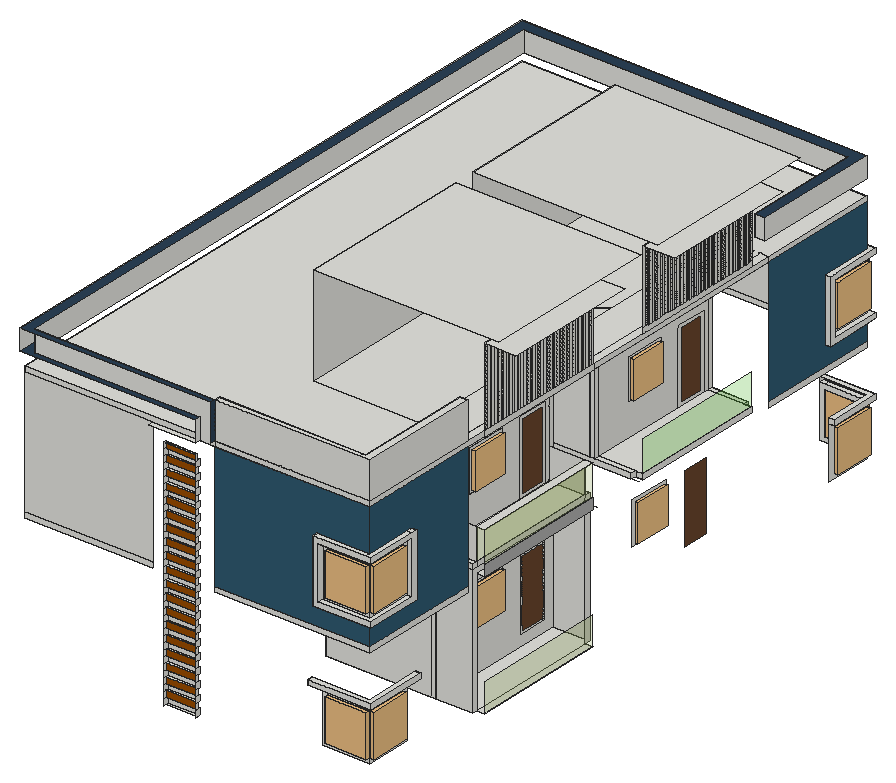
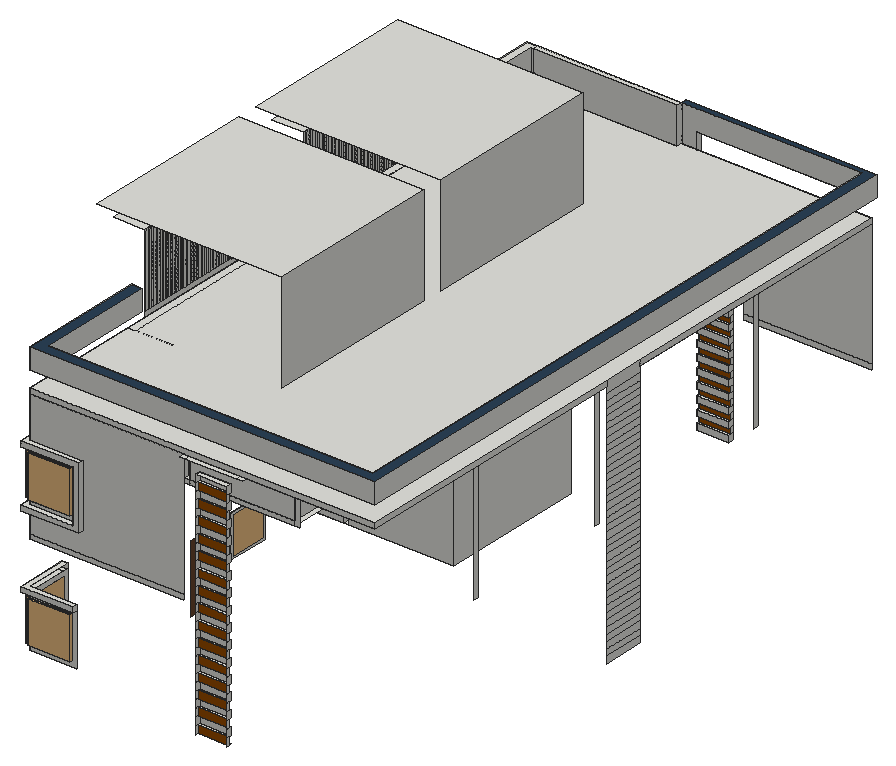
# SketchUp Ruby script. Lengths in inches.
U = 1.inch
M = Sketchup.active_model
def pt(a) = Geom::Point3d.new(a.map { |v| v * U })
def face(e, loops, mat)
  f = e.add_face(loops[0].map { |a| pt(a) })
  loops[1..].each { |l| e.add_face(l.map { |a| pt(a) }).erase! }
  f.material = f.back_material = mat if mat
  f
end
# faces: each face lists its corners as indices into pts; further lists are holes
def faces(e, pts, list, mat = nil) = list.each { |f| face(e, (f[0].is_a?(Array) ? f : [f]).map { |l| l.map { |i| pts[i] } }, mat) }
# xy, xz, yz: faces in a plane at the given z, y or x. An outline is a flat list of corners, or four numbers for a rectangle; further outlines are holes
def ring(l) = l.size == 4 ? [[l[0], l[1]], [l[2], l[1]], [l[2], l[3]], [l[0], l[3]]] : l.each_slice(2).to_a
def flat(e, list, mat, &to3) = list.each { |f| face(e, (f[0].is_a?(Array) ? f : [f]).map { |l| ring(l).map { |u, v| to3.(u, v) } }, mat) }
def xy(e, z, list, mat = nil) = flat(e, list, mat) { |x, y| [x, y, z] }
def xz(e, y, list, mat = nil) = flat(e, list, mat) { |x, z| [x, y, z] }
def yz(e, x, list, mat = nil) = flat(e, list, mat) { |y, z| [x, y, z] }
def lines(e, pts, list) = list.each { |a, b| e.add_line(pt(pts[a]), pt(pts[b])) }
# prism: a flat outline (further loops are holes) pulled along v
def prism(e, loops, v, mat = nil)
  f = face(e, loops, mat); d = Geom::Vector3d.new(v.map { |x| x * U })
  f.pushpull(f.normal.samedirection?(d) ? d.length : -d.length)
end
def box(e, o, s, mat = nil) = prism(e, [[o, [o[0] + s[0], o[1], o[2]], [o[0] + s[0], o[1] + s[1], o[2]], [o[0], o[1] + s[1], o[2]]]], [0, 0, s[2]], mat)
def at(x, y, z, deg = 0) = Geom::Transformation.translation(pt([x, y, z])) * Geom::Transformation.rotation(ORIGIN, Z_AXIS, deg.degrees)
def axes(o, x, y, z) = Geom::Transformation.new([*x, 0, *y, 0, *z, 0, *pt(o).to_a, 1])
def part(name) = M.definitions.add(name)
# library, detail: a bought-in or finely detailed component or shape, given as its bounding box
def library(name, o, s) = part(name).tap { |d| box(d.entities, o, s) }
def detail(e, o, s) = box(e.add_group.entities, o, s)
def put(e, d, t, mat = nil) = e.add_instance(d, t).tap { |i| i.material = mat if mat }
def group(e, t, mat = nil) = e.add_group.tap { |g| g.transformation = t; g.material = mat if mat }.entities
root = M.entities
M.materials.add("C07_Caramel_Shine").color = [153, 76, 0]
M.materials.add("Carpet_04_1K").color = [43, 65, 85]
M.materials.add("Glass_Basic_01").color = [173, 201, 98]
M.materials["Glass_Basic_01"].alpha = 0.25
M.materials.add("Glass_Basic_2").color = [93, 234, 42]
M.materials["Glass_Basic_2"].alpha = 0.25
M.materials.add("ThomThom - Jumper1").color = [47, 89, 112]
M.materials.add("ThomThom - Waistcoat2").color = [170, 170, 169]
M.materials.add("Wood_Veneer_15_1K").color = [103, 69, 45]
c1 = library("Group\#5",[0,0,0],[1.97,28.21,60])
xy(root,453,[[435,495,555,663],[555,495,561,663],[561,495,603,663],[603,501,612,657]])
xy(root,455.25,[[381,333,417,336]])
xy(root,458.25,[[381,1050,417,1053]])
xy(root,462.375,[[381,333,417,336]])
xy(root,467.17,[[381,1050,417,1053]])
xy(root,469.5,[[381,333,417,336]])
xy(root,476.1,[[381,1050,417,1053]])
xy(root,476.625,[[381,333,417,336]])
xy(root,483.75,[[381,333,417,336]])
xy(root,485.02,[[381,1050,417,1053]])
xy(root,490.875,[[381,333,417,336]])
xy(root,493.95,[[381,1050,417,1053]])
xy(root,498,[[381,333,417,336]])
xy(root,502.875,[[381,1050,417,1053]])
xy(root,505.125,[[381,333,417,336]])
xy(root,511.8,[[381,1050,417,1053]])
xy(root,512.25,[[381,333,417,336]])
xy(root,519.375,[[381,333,417,336]])
xy(root,520.72,[[381,1050,417,1053]])
xy(root,526.5,[[381,333,417,336]])
xy(root,529.65,[[381,1050,417,1053]])
xy(root,533.625,[[381,333,417,336]])
xy(root,534,[[546,330,558,336],[558,330,618,336],[612,336,618,390],[612,390,618,402],[612,996,618,1002],
  [612,1002,618,1056],[557.39,1050,564.01,1056],[564.01,1050,612,1056]])
xy(root,538.57,[[381,1050,417,1053]])
xy(root,540,[[546,330,618,330,618,402,612,402,612,336,546,336],[612,996,612,1050,557.39,1050,557.39,1056,618,1056,618,996]])
xy(root,540.75,[[381,333,417,336]])
xy(root,547.5,[[381,1050,417,1053]])
xy(root,547.875,[[381,333,417,336]])
xy(root,555,[[381,333,417,336]])
xy(root,556.42,[[381,1050,417,1053]])
xy(root,562.125,[[381,333,417,336]])
xy(root,565.35,[[381,1050,417,1053]])
xy(root,569.25,[[381,333,417,336]])
xy(root,574.27,[[381,1050,417,1053]])
xy(root,576.375,[[381,333,417,336]])
xy(root,583.2,[[381,1050,417,1053]])
xy(root,583.5,[[381,333,417,336]])
xy(root,590.625,[[381,333,417,336]])
xy(root,592.125,[[381,1050,417,1053]])
xy(root,593.66,[[435,723,555,891],[555,723,561,891],[561,723,603,723,603,729,612,729,612,885,603,885,603,891,561,891]])
xy(root,594,[[603,501,612,657]])
xy(root,597.75,[[381,333,417,336]])
xy(root,599.66,[[435,723,555,891],[555,723,561,891],[561,723,603,729],[561,729,612,885],[561,885,603,891]])
xy(root,600,[[435,495,555,663],[555,495,561,663],[561,495,603,663]])
xy(root,601.05,[[381,1050,417,1053]])
xy(root,602.66,[[555,846,561,876]])
xy(root,604.875,[[381,333,417,336]])
xy(root,606,[[435,495,555,663],[555,495,561,663],[561,495,603,501],[561,501,603,657],[561,657,603,663]])
xy(root,609,[[555,618,561,648]])
xy(root,609.97,[[381,1050,417,1053]])
xy(root,612,[[381,333,417,336]])
xy(root,618,[[552,330,558,336],[558,330,612,336],[612,330,618,390],[612,390,618,396],[612,990,618,1050],
  [551.39,1050,618,1056]])
xy(root,618.9,[[381,1050,417,1053]])
xy(root,619.125,[[381,333,417,336]])
xy(root,624,[[558,330,618,330,618,390,612,390,612,336,558,336],[612,996,612,1050,557.39,1050,557.39,1056,618,1056,618,996]])
xy(root,626.25,[[381,333,417,336]])
xy(root,627.83,[[381,1050,417,1053]])
xy(root,633.375,[[381,333,417,336]])
xy(root,636.75,[[381,1050,417,1053]])
xy(root,638.66,[[555,774,561,816]])
xy(root,640.5,[[381,333,417,336]])
xy(root,642,[[603,501,612,657]])
xy(root,645,[[555,546,561,588]])
xy(root,645.67,[[381,1050,417,1053]])
xy(root,647.625,[[381,333,417,336]])
xy(root,654.6,[[381,1050,417,1053]])
xy(root,654.75,[[381,333,417,336]])
xy(root,661.875,[[381,333,417,336]])
xy(root,663.52,[[381,1050,417,1053]])
xy(root,669,[[381,333,417,336]])
xy(root,672.45,[[381,1050,417,1053]])
xy(root,676.125,[[381,333,417,336]])
xy(root,680.66,[[555,774,561,816],[555,846,561,876]])
xy(root,681.375,[[381,1050,417,1053]])
xy(root,683.25,[[381,333,417,336]])
xy(root,684,[[558,330,558,336,612,336,612,390,618,390,618,330],[612,996,618,996,618,1056,557.39,1056,557.39,1050,612,1050]])
xy(root,687,[[555,546,561,588],[555,618,561,648]])
xy(root,690,[[552,330,612,336],[612,330,618,390],[612,390,618,396],[612,990,612,1050,551.39,1050,551.39,1056,618,1056,618,990]])
xy(root,690.3,[[381,1050,417,1053]])
xy(root,690.375,[[381,333,417,336]])
xy(root,697.5,[[381,333,417,336]])
xy(root,699.22,[[381,1050,417,1053]])
xy(root,704.625,[[381,333,417,336]])
xy(root,708.15,[[381,1050,417,1053]])
xy(root,711.75,[[381,333,417,336]])
xy(root,717.08,[[381,1050,417,1053]])
xy(root,718.875,[[381,332.4,417,336]])
xy(root,726,[[381,330,417,332.4],[381,1050,417,1056]])
xy(root,738,[[363,330,369,330,369,489,429,489,429,345,369,345,369,330,417,330,417,336,435,336,435,489,561,489,561,495,225,495,225,489,363,489],[216,336,363,336,363,345,225,345,225,669,216,669],[216,336,612,1050],[435,336,612,336,612,477,561,477,561,345,435,345],[429,495,435,495,435,663,555,663,555,495,561,495,561,669,225,669,225,663,429,663],
  [561,501,613,657],[216,717,216,1050,363,1050,363,1041,225,1041,225,717],[225,717,225,723,429,723,429,891,435,891,435,723,561,723,561,717],[555,723,555,891,225,891,225,897,363,897,363,1056,369,1056,369,897,429,897,429,1056,435,1056,435,897,561,897,561,723],[561,909,561,1041,435,1041,435,1050,612,1050,612,909],
  [369,1041,429,1056]])
xy(root,743.66,[[561,729,612,885]])
xy(root,744,[[216,336,612,336,612,477,602.94,477,602.94,909,612,909,612,1050,216,1050],[435,336,600,342],[600,336,600,342,603,342,603,477,612,477,612,336],[435,477,561,681],[602.94,477,612,909],
  [612,501,613,657],[435,705,561,909]])
xy(root,762,[[216,330,216,1050,612,1050,612,903.7,600,903.7,600,1038,228,1038,228,336,417,336,417,330]],"Carpet_04_1K")
xy(root,786,[[435,336,600,342],[600,336,612,336,612,477,603,477,603,342,600,342]])
xy(root,786,[[216,330,435,330,435,336,228,336,228,1038,600,1038,600,903.7,612,903.7,612,1050,216,1050]],"Carpet_04_1K")
xy(root,834,[[612,501,648,657],[612,729,648,885]])
xy(root,858,[[435,477,648,681],[435,705,648,909]])
xz(root,330,[[546,534,618,540],[552,618,618,618,618,624,558,624,558,684,618,684,618,690,552,690]])
xz(root,332.4,[[381,718.875,417,726]],"C07_Caramel_Shine")
xz(root,333,[[381,462.375,417,469.5],[381,476.625,417,483.75],[381,490.875,417,498],[381,505.125,417,512.25],[381,519.375,417,526.5],
  [381,533.625,417,540.75],[381,547.875,417,555],[381,562.125,417,569.25],[381,576.375,417,583.5],[381,590.625,417,597.75],
  [381,604.875,417,612],[381,619.125,417,626.25],[381,633.375,417,640.5],[381,647.625,417,654.75],[381,661.875,417,669],
  [381,676.125,417,683.25],[381,690.375,417,697.5],[381,704.625,417,711.75]],"C07_Caramel_Shine")
xz(root,336,[[381,455.25,417,462.375],[381,469.5,417,476.625],[558,474,612,474,612,480,564,480,564,528,612,528,612,534,558,534],[564,480,612,528],[381,483.75,417,490.875],
  [381,498,417,505.125],[381,512.25,417,519.375],[381,526.5,417,533.625],[381,540.75,417,547.875],[381,555,417,562.125],
  [381,569.25,417,576.375],[381,583.5,417,590.625],[216,588,363,594],[435,588,612,594],[216,594,363,738],
  [381,597.75,417,604.875],[381,612,417,619.125],[558,624,612,624,612,630,564,630,564,678,612,678,612,684,558,684],[381,626.25,417,633.375],[564,630,612,678],
  [381,640.5,417,647.625],[381,654.75,417,661.875],[381,669,417,676.125],[381,683.25,417,690.375],[381,697.5,417,704.625],
  [381,711.75,417,718.875],[216,738,612,744],[417,738,417,762,228,762,228,786,435,786,435,738],[435,744,612,786]])
xz(root,336,[[435,594,612,594,612,618,552,618,552,690,612,690,612,738,435,738]],"ThomThom - Jumper1")
xz(root,342,[[435,744,600,786],[600,744,603,786]])
xz(root,390,[[612,624,618,684]])
xz(root,396,[[612,618,618,624],[612,624,618,684],[612,684,618,690]])
xz(root,402,[[612,534,618,540]])
xz(root,477,[[602.94,744,603,786],[603,744,612,786]])
xz(root,495,[[435,453,555,600],[555,453,561,600],[561,453,603,600],[429,594,435,738],[435,600,603,606],
  [435,606,555,738],[555,606,561,738]])
xz(root,501,[[561,606,603,642]])
xz(root,546,[[555,645,561,687]])
xz(root,588,[[555,645,561,687]])
xz(root,618,[[555,609,561,687]])
xz(root,648,[[555,609,561,687]])
xz(root,657,[[561,606,603,642]])
xz(root,663,[[435,453,555,600],[561,453,603,600],[435,600,555,606],[555,600,561,606],[561,600,603,606],
  [435,606,555,738]])
xz(root,723,[[435,593.66,603,599.66],[435,599.66,555,738],[555,599.66,561,738]])
xz(root,729,[[603,593.66,612,599.66]])
xz(root,774,[[555,638.66,561,680.66]])
xz(root,816,[[555,638.66,561,680.66]])
xz(root,846,[[555,602.66,561,680.66]])
xz(root,876,[[555,602.66,561,680.66]])
xz(root,885,[[603,593.66,612,599.66]])
xz(root,891,[[435,593.66,555,599.66],[555,593.66,561,599.66],[561,593.66,603,599.66],[429,594,435,738],[435,599.66,555,738]])
xz(root,903.7,[[600,762,612,786]])
xz(root,909,[[561,738,612,744]])
xz(root,990,[[612,618,618,690]])
xz(root,996,[[612,534,618,540],[612,624,618,684]])
xz(root,1038,[[228,762,600,786]])
xz(root,1050,[[381,467.17,417,476.1],[557.39,474,612,474,612,480,564.01,480,564.01,528,612,528,612,534,557.39,534],[564.01,480,612,528],[381,485.02,417,493.95],[381,502.875,417,511.8],
  [381,520.72,417,529.65],[381,538.57,417,547.5],[381,556.42,417,565.35],[381,574.27,417,583.2],[435,588,612,594],
  [381,592.125,417,601.05],[435,594,612,594,612,618,551.39,618,551.39,690,612,690,612,738,435,738],[381,609.97,417,618.9],[557.39,624,612,624,612,630,564.01,630,564.01,678,612,678,612,684,557.39,684],[381,627.83,417,636.75],
  [564.01,630,612,678],[381,645.67,417,654.6],[381,663.52,417,672.45],[381,681.375,417,690.3],[381,699.22,417,708.15],
  [381,717.08,417,726],[216,738,612,744],[216,762,612,786]])
xz(root,1053,[[381,458.25,417,467.17],[381,476.1,417,485.02],[381,493.95,417,502.875],[381,511.8,417,520.72],[381,529.65,417,538.57],
  [381,547.5,417,556.42],[381,565.35,417,574.27],[381,583.2,417,592.125],[381,601.05,417,609.97],[381,618.9,417,627.83],
  [381,636.75,417,645.67],[381,654.6,417,663.52],[381,672.45,417,681.375],[381,690.3,417,699.22],[381,708.15,417,717.08]],"C07_Caramel_Shine")
xz(root,1056,[[557.39,534,618,540],[551.39,618,618,618,618,624,557.39,624,557.39,684,618,684,618,690,551.39,690]])
yz(root,216,[[669,453,717,460.5],[669,460.5,717,468],[669,468,717,475.5],[669,475.5,717,483],[669,483,717,490.5],
  [669,490.5,717,498],[669,498,717,505.5],[669,505.5,717,513],[669,513,717,520.5],[669,520.5,717,528],
  [669,528,717,535.5],[669,535.5,717,543],[669,543,717,550.5],[669,550.5,717,558],[669,558,717,565.5],
  [669,565.5,717,573],[669,573,717,580.5],[669,580.5,717,588],[669,588,717,595.5],[669,595.5,717,603],
  [669,603,717,610.5],[669,610.5,717,618],[669,618,717,625.5],[669,625.5,717,633],[669,633,717,640.5],
  [669,640.5,717,648],[669,648,717,655.5],[669,655.5,717,663],[669,663,717,670.5],[669,670.5,717,678],
  [669,678,717,685.5],[669,685.5,717,693],[669,693,717,700.5],[669,700.5,717,708],[669,708,717,715.5],
  [669,715.5,717,723],[669,723,717,730.5],[669,730.5,717,744],[336,738,669,744],[717,738,1050,744],
  [330,762,1050,786]])
yz(root,225,[[489,594,495,738],[663,594,669,738],[717,594,723,738],[891,594,897,738]])
yz(root,228,[[336,762,1038,786]])
yz(root,381,[[330,455.25,336,462.375],[1053,458.25,1056,467.17],[330,462.375,333,469.5],[1050,467.17,1056,476.1],[330,469.5,336,476.625],
  [1053,476.1,1056,485.02],[330,476.625,333,483.75],[330,483.75,336,490.875],[1050,485.02,1056,493.95],[330,490.875,333,498],
  [1053,493.95,1056,502.875],[330,498,336,505.125],[1050,502.875,1056,511.8],[330,505.125,333,512.25],[1053,511.8,1056,520.72],
  [330,512.25,336,519.375],[330,519.375,333,526.5],[1050,520.72,1056,529.65],[330,526.5,336,533.625],[1053,529.65,1056,538.57],
  [330,533.625,333,540.75],[1050,538.57,1056,547.5],[330,540.75,336,547.875],[1053,547.5,1056,556.42],[330,547.875,333,555],
  [330,555,336,562.125],[1050,556.42,1056,565.35],[330,562.125,333,569.25],[1053,565.35,1056,574.27],[330,569.25,336,576.375],
  [1050,574.27,1056,583.2],[330,576.375,333,583.5],[1053,583.2,1056,592.125],[330,583.5,336,590.625],[330,590.625,333,597.75],
  [1050,592.125,1056,601.05],[330,597.75,336,604.875],[1053,601.05,1056,609.97],[330,604.875,333,612],[1050,609.97,1056,618.9],
  [330,612,336,619.125],[1053,618.9,1056,627.83],[330,619.125,333,626.25],[330,626.25,336,633.375],[1050,627.83,1056,636.75],
  [330,633.375,333,640.5],[1053,636.75,1056,645.67],[330,640.5,336,647.625],[1050,645.67,1056,654.6],[330,647.625,333,654.75],
  [1053,654.6,1056,663.52],[330,654.75,336,661.875],[330,661.875,333,669],[1050,663.52,1056,672.45],[330,669,336,676.125],
  [1053,672.45,1056,681.375],[330,676.125,333,683.25],[1050,681.375,1056,690.3],[330,683.25,336,690.375],[1053,690.3,1056,699.22],
  [330,690.375,333,697.5],[330,697.5,336,704.625],[1050,699.22,1056,708.15],[330,704.625,333,711.75],[1053,708.15,1056,717.08],
  [330,711.75,336,718.875],[1050,717.08,1056,726],[330,718.875,332.4,726]])
yz(root,417,[[330,455.25,336,462.375],[1053,458.25,1056,467.17],[330,462.375,333,469.5],[1050,467.17,1056,476.1],[330,469.5,336,476.625],
  [1053,476.1,1056,485.02],[330,476.625,333,483.75],[330,483.75,336,490.875],[1050,485.02,1056,493.95],[330,490.875,333,498],
  [1053,493.95,1056,502.875],[330,498,336,505.125],[1050,502.875,1056,511.8],[330,505.125,333,512.25],[1053,511.8,1056,520.72],
  [330,512.25,336,519.375],[330,519.375,333,526.5],[1050,520.72,1056,529.65],[330,526.5,336,533.625],[1053,529.65,1056,538.57],
  [330,533.625,333,540.75],[1050,538.57,1056,547.5],[330,540.75,336,547.875],[1053,547.5,1056,556.42],[330,547.875,333,555],
  [330,555,336,562.125],[1050,556.42,1056,565.35],[330,562.125,333,569.25],[1053,565.35,1056,574.27],[330,569.25,336,576.375],
  [1050,574.27,1056,583.2],[330,576.375,333,583.5],[1053,583.2,1056,592.125],[330,583.5,336,590.625],[330,590.625,333,597.75],
  [1050,592.125,1056,601.05],[330,597.75,336,604.875],[1053,601.05,1056,609.97],[330,604.875,333,612],[1050,609.97,1056,618.9],
  [330,612,336,619.125],[1053,618.9,1056,627.83],[330,619.125,333,626.25],[330,626.25,336,633.375],[1050,627.83,1056,636.75],
  [330,633.375,333,640.5],[1053,636.75,1056,645.67],[330,640.5,336,647.625],[1050,645.67,1056,654.6],[330,647.625,333,654.75],
  [1053,654.6,1056,663.52],[330,654.75,336,661.875],[330,661.875,333,669],[1050,663.52,1056,672.45],[330,669,336,676.125],
  [1053,672.45,1056,681.375],[330,676.125,333,683.25],[1050,681.375,1056,690.3],[330,683.25,336,690.375],[1053,690.3,1056,699.22],
  [330,690.375,333,697.5],[330,697.5,336,704.625],[1050,699.22,1056,708.15],[330,704.625,333,711.75],[1053,708.15,1056,717.08],
  [330,711.75,336,718.875],[1050,717.08,1056,726],[330,718.875,332.4,726],[330,738,336,762]])
yz(root,435,[[495,453,663,600],[723,599.66,891,738],[495,600,663,606],[495,606,663,738],[336,744,342,786],
  [477,744,681,858],[705,744,909,858]])
yz(root,435,[[330,744,336,786]],"Carpet_04_1K")
yz(root,546,[[330,534,336,540]])
yz(root,551.39,[[1050,618,1056,690]])
yz(root,552,[[330,618,336,624],[330,624,336,684],[330,684,336,690]])
yz(root,555,[[495,594,663,600],[[723,599.66,891,738],[846,602.66,876,680.66],[774,638.66,816,680.66]],[[495,606,663,738],[618,609,648,687],[546,645,588,687]]])
yz(root,557.39,[[1050,534,1056,540],[1050,624,1056,684]])
yz(root,558,[[330,624,336,684]])
yz(root,561,[[[495,453,663,594],[615,465.34,651,549.34],[543,501.34,591,549.34]],[[615,465.34,651,549.34],[618,468.34,648,546.34]],[[777,485.66,825,533.66],[780,488.66,822,530.66]],[[543,501.34,591,549.34],[546,504.34,588,546.34]],[495,594,663,600],
  [723,599.66,729,738],[[729,599.66,729,738,885,738,885,599.66,879,599.66,879,683.66,843,683.66,843,599.66],[771,635.66,819,683.66]],[[843,599.66,879,683.66],[846,602.66,876,680.66]],[885,599.66,891,738],[495,606,501,738],
  [[501,606,615,606,615,690,651,690,651,606,657,606,657,738,501,738],[543,642,591,690]],[[615,606,651,690],[618,609,648,687]],[657,606,663,738],[[771,635.66,819,683.66],[774,638.66,816,680.66]],[[543,642,591,690],[546,645,588,687]]])
yz(root,561,[[852,452.66,882,530.66],[618,468.34,648,546.34],[846,602.66,876,680.66],[618,609,648,687]],"Wood_Veneer_15_1K")
yz(root,600,[[903.7,762,1038,786]])
yz(root,603,[[495,453,495,600,663,600,663,453,657,453,657,594,501,594,501,453],[723,593.66,729,599.66],[885,593.66,891,599.66],[495,600,501,606],[501,600,657,606],
  [657,600,663,606],[342,744,477,786]])
yz(root,603,[[501,606,657,642]],"Glass_Basic_01")
yz(root,612,[[336,474,390,474,390,534,336,534,336,528,384,528,384,480,336,480],[996,474,996,534,1050,534,1050,528,1002,528,1002,480,1050,480,1050,474],[336,480,384,528],[1002,480,1050,528],[336,588,477,594],
  [909,588,1050,594],[729,593.66,885,599.66],[336,624,390,624,390,684,336,684,336,678,384,678,384,630,336,630],[996,624,996,684,1050,684,1050,678,1002,678,1002,630,1050,630,1050,624],[336,630,384,678],
  [1002,630,1050,678],[336,738,909,744],[909,738,1050,744],[729,743.66,885,749.66],[336,744,477,786],
  [501,744,503.6,834],[503.6,744,506.2,834],[506.2,744,508.8,834],[508.8,744,511.4,834],[511.4,744,514,834],
  [514,744,516.6,834],[516.6,744,519.2,834],[519.2,744,521.8,834],[521.8,744,524.4,834],[524.4,744,527,834],
  [527,744,529.6,834],[529.6,744,532.2,834],[532.2,744,534.8,834],[534.8,744,537.4,834],[537.4,744,540,834],
  [540,744,542.6,834],[542.6,744,545.2,834],[545.2,744,547.8,834],[547.8,744,550.4,834],[550.4,744,553,834],
  [553,744,555.6,834],[555.6,744,558.2,834],[558.2,744,560.8,834],[560.8,744,563.4,834],[563.4,744,566,834],
  [566,744,568.6,834],[568.6,744,571.2,834],[571.2,744,573.8,834],[573.8,744,576.4,834],[576.4,744,579,834],
  [579,744,581.6,834],[581.6,744,584.2,834],[584.2,744,586.8,834],[586.8,744,589.4,834],[589.4,744,592,834],
  [592,744,594.6,834],[594.6,744,597.2,834],[597.2,744,599.8,834],[599.8,744,602.4,834],[602.4,744,605,834],
  [605,744,607.6,834],[607.6,744,610.2,834],[610.2,744,612.8,834],[612.8,744,615.4,834],[615.4,744,618,834],
  [618,744,620.6,834],[620.6,744,623.2,834],[623.2,744,625.8,834],[625.8,744,628.4,834],[628.4,744,631,834],
  [631,744,633.6,834],[633.6,744,636.2,834],[636.2,744,638.8,834],[638.8,744,641.4,834],[641.4,744,644,834],
  [644,744,646.6,834],[646.6,744,649.2,834],[649.2,744,651.8,834],[651.8,744,654.4,834],[654.4,744,657,834],
  [729,749.66,730.95,834],[730.95,749.66,732.9,834],[732.9,749.66,734.85,834],[734.85,749.66,736.8,834],[736.8,749.66,738.75,834],
  [738.75,749.66,740.7,834],[740.7,749.66,742.65,834],[742.65,749.66,744.6,834],[744.6,749.66,746.55,834],[746.55,749.66,748.5,834],
  [748.5,749.66,750.45,834],[750.45,749.66,752.4,834],[752.4,749.66,754.35,834],[754.35,749.66,756.3,834],[756.3,749.66,758.25,834],
  [758.25,749.66,760.2,834],[760.2,749.66,762.15,834],[762.15,749.66,764.1,834],[764.1,749.66,766.05,834],[766.05,749.66,768,834],
  [768,749.66,769.95,834],[769.95,749.66,771.9,834],[771.9,749.66,773.85,834],[773.85,749.66,775.8,834],[775.8,749.66,777.75,834],
  [777.75,749.66,779.7,834],[779.7,749.66,781.65,834],[781.65,749.66,783.6,834],[783.6,749.66,785.55,834],[785.55,749.66,787.5,834],
  [787.5,749.66,789.45,834],[789.45,749.66,791.4,834],[791.4,749.66,793.35,834],[793.35,749.66,795.3,834],[795.3,749.66,797.25,834],
  [797.25,749.66,799.2,834],[799.2,749.66,801.15,834],[801.15,749.66,803.1,834],[803.1,749.66,805.05,834],[805.05,749.66,807,834],
  [807,749.66,808.95,834],[808.95,749.66,810.9,834],[810.9,749.66,812.85,834],[812.85,749.66,814.8,834],[814.8,749.66,816.75,834],
  [816.75,749.66,818.7,834],[818.7,749.66,820.65,834],[820.65,749.66,822.6,834],[822.6,749.66,824.55,834],[824.55,749.66,826.5,834],
  [826.5,749.66,828.45,834],[828.45,749.66,830.4,834],[830.4,749.66,832.35,834],[832.35,749.66,834.3,834],[834.3,749.66,836.25,834],
  [836.25,749.66,838.2,834],[838.2,749.66,840.15,834],[840.15,749.66,842.1,834],[842.1,749.66,844.05,834],[844.05,749.66,846,834],
  [846,749.66,847.95,834],[847.95,749.66,849.9,834],[849.9,749.66,851.85,834],[851.85,749.66,853.8,834],[853.8,749.66,855.75,834],
  [855.75,749.66,857.7,834],[857.7,749.66,859.65,834],[859.65,749.66,861.6,834],[861.6,749.66,863.55,834],[863.55,749.66,865.5,834],
  [865.5,749.66,867.45,834],[867.45,749.66,869.4,834],[869.4,749.66,871.35,834],[871.35,749.66,873.3,834],[873.3,749.66,875.25,834],
  [875.25,749.66,877.2,834],[877.2,749.66,879.15,834],[879.15,749.66,881.1,834],[881.1,749.66,883.05,834],[883.05,749.66,885,834],
  [903.7,762,1050,786]])
yz(root,612,[[501,453,657,486],[501,606,657,642]],"Glass_Basic_01")
yz(root,612,[[729,599.66,885,635.66]],"Glass_Basic_2")
yz(root,612,[[336,594,477,594,477,738,336,738,336,690,396,690,396,618,336,618],[909,594,909,738,1050,738,1050,690,990,690,990,618,1050,618,1050,594]],"ThomThom - Jumper1")
yz(root,612,[[501,594,657,606]],"ThomThom - Waistcoat2")
yz(root,613,[[501,738,657,744]])
yz(root,618,[[330,534,402,540],[996,534,1056,540],[330,618,396,618,396,690,330,690,330,684,390,684,390,624,330,624],[990,618,990,690,1056,690,1056,684,996,684,996,624,1056,624,1056,618]])
p = [[561,543,642],[561,591,642],[561,591,690],[561,543,690],[603,663,594],[612,663,594],
  [602.94,681,744],[602.94,477,744],[603,681,744],[603,723,594],[612,723,594]]
lines(root,p,[[0,1],[1,2],[2,3],[3,0],[4,5],[6,7],[7,8],[9,10]])
put(root,c1,axes([616.44,1050,479.94],[-2.50681,0,0],[0,-1.70151,0],[0,0,0.801]))
put(root,c1,axes([564,331.56,479.94],[0,2.50681,0],[1.70151,0,0],[0,0,0.801]))
put(root,c1,axes([616.93,336,480],[-2.50681,0,0],[0,1.70151,0],[0,0,0.801]))
put(root,c1,axes([564.04,1052.45,480.01],[0,-1.3838,0],[1.7,0,0],[0,0,0.7998]))
put(root,c1,axes([565.44,822,488.66],[-2.50681,0,0],[0,-1.48882,0],[0,0,0.70007]))
put(root,c1,axes([565.93,546,504.34],[-2.50681,0,0],[0,1.48882,0],[0,0,0.70007]))
put(root,c1,axes([616.44,1050,629.94],[-2.50681,0,0],[0,-1.70151,0],[0,0,0.801]))
put(root,c1,axes([564,331.56,629.94],[0,2.50681,0],[1.70151,0,0],[0,0,0.801]))
put(root,c1,axes([616.93,336,630],[-2.50681,0,0],[0,1.70151,0],[0,0,0.801]))
put(root,c1,axes([564.04,1052.45,630.01],[0,-1.3838,0],[1.7,0,0],[0,0,0.7998]))
put(root,c1,axes([565.44,816,638.66],[-2.50681,0,0],[0,-1.48882,0],[0,0,0.70007]))
put(root,c1,axes([565.93,546,645],[-2.50681,0,0],[0,1.48882,0],[0,0,0.70007]))
